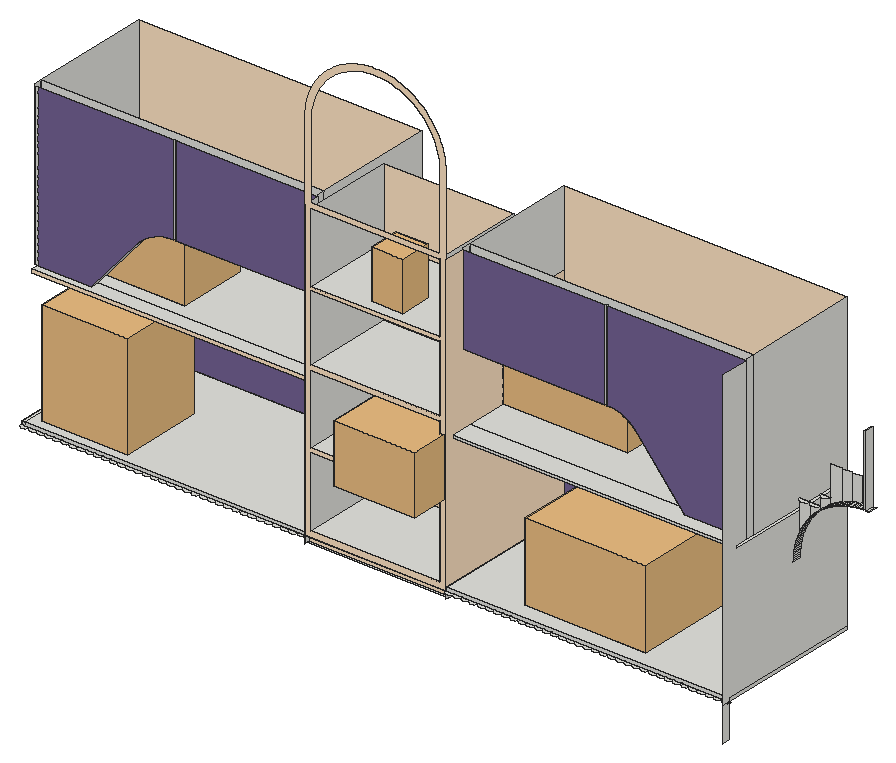
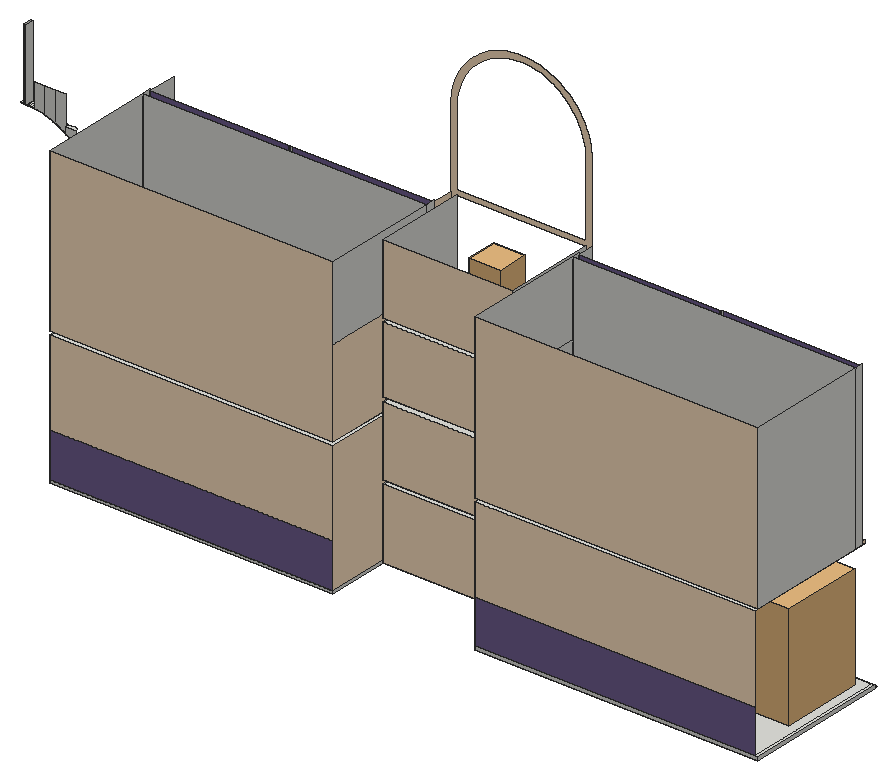
# SketchUp Ruby script. Lengths in inches.
U = 1.inch
M = Sketchup.active_model
def pt(a) = Geom::Point3d.new(a.map { |v| v * U })
def face(e, loops, mat)
  f = e.add_face(loops[0].map { |a| pt(a) })
  loops[1..].each { |l| e.add_face(l.map { |a| pt(a) }).erase! }
  f.material = f.back_material = mat if mat
  f
end
# faces: each face lists its corners as indices into pts; further lists are holes
def faces(e, pts, list, mat = nil) = list.each { |f| face(e, (f[0].is_a?(Array) ? f : [f]).map { |l| l.map { |i| pts[i] } }, mat) }
# xy, xz, yz: faces in a plane at the given z, y or x. An outline is a flat list of corners, or four numbers for a rectangle; further outlines are holes
def ring(l) = l.size == 4 ? [[l[0], l[1]], [l[2], l[1]], [l[2], l[3]], [l[0], l[3]]] : l.each_slice(2).to_a
def flat(e, list, mat, &to3) = list.each { |f| face(e, (f[0].is_a?(Array) ? f : [f]).map { |l| ring(l).map { |u, v| to3.(u, v) } }, mat) }
def xy(e, z, list, mat = nil) = flat(e, list, mat) { |x, y| [x, y, z] }
def xz(e, y, list, mat = nil) = flat(e, list, mat) { |x, z| [x, y, z] }
def yz(e, x, list, mat = nil) = flat(e, list, mat) { |y, z| [x, y, z] }
def lines(e, pts, list) = list.each { |a, b| e.add_line(pt(pts[a]), pt(pts[b])) }
# prism: a flat outline (further loops are holes) pulled along v
def prism(e, loops, v, mat = nil)
  f = face(e, loops, mat); d = Geom::Vector3d.new(v.map { |x| x * U })
  f.pushpull(f.normal.samedirection?(d) ? d.length : -d.length)
end
def box(e, o, s, mat = nil) = prism(e, [[o, [o[0] + s[0], o[1], o[2]], [o[0] + s[0], o[1] + s[1], o[2]], [o[0], o[1] + s[1], o[2]]]], [0, 0, s[2]], mat)
def at(x, y, z, deg = 0) = Geom::Transformation.translation(pt([x, y, z])) * Geom::Transformation.rotation(ORIGIN, Z_AXIS, deg.degrees)
def axes(o, x, y, z) = Geom::Transformation.new([*x, 0, *y, 0, *z, 0, *pt(o).to_a, 1])
def part(name) = M.definitions.add(name)
# library, detail: a bought-in or finely detailed component or shape, given as its bounding box
def library(name, o, s) = part(name).tap { |d| box(d.entities, o, s) }
def detail(e, o, s) = box(e.add_group.entities, o, s)
def put(e, d, t, mat = nil) = e.add_instance(d, t).tap { |i| i.material = mat if mat }
def group(e, t, mat = nil) = e.add_group.tap { |g| g.transformation = t; g.material = mat if mat }.entities
root = M.entities
M.materials.add("[0012_Bisque]").color = [255, 228, 196]
M.materials.add("[Color I01]").color = [116, 98, 147]
c1 = library("Flower+Vase+Glass",[1.07,1.25,0],[13.84,13.38,16.78])
c2 = library("Architecture and design books\#1",[9.67,-0.02,0],[20.02,11.1,12.25])
c3 = library("Group\#3",[0,0,0],[2.77,2.73,4.26])
c4 = library("pen_stand",[0,-5.91,0],[13.07,11.82,9.49])
c5 = library("LapTop",[-9.12,-3.35,-0.68],[14.19,15.07,9.17])
xy(root,39.45,[[50.74,141.7,73.56,142.13]])
xy(root,40.6875,[[5.77,140.54,5.94,140.5625,6.1,140.63,6.24,140.73,6.34,140.87,6.41,141.03,6.43,141.2,5.12,141.2,5.14,141.03,5.2,140.87,5.31,140.73,5.44,140.63,5.6,140.5625],[7.08,140.54,7.25,140.5625,7.41,140.63,7.55,140.73,7.65,140.87,7.72,141.03,7.74,141.2,6.43,141.2,6.45,141.03,6.52,140.87,6.62,140.73,6.76,140.63,6.91,140.5625],[8.4,140.54,8.57,140.5625,8.72,140.63,8.86,140.73,8.96,140.87,9.03,141.03,9.05,141.2,7.74,141.2,7.76,141.03,7.83,140.87,7.93,140.73,8.07,140.63,8.23,140.5625],[9.71,140.54,9.88,140.5625,10.04,140.63,10.17,140.73,10.28,140.87,10.34,141.03,10.37,141.2,9.05,141.2,9.08,141.03,9.14,140.87,9.24,140.73,9.38,140.63,9.54,140.5625],[11.02,140.54,11.19,140.5625,11.35,140.63,11.49,140.73,11.59,140.87,11.66,141.03,11.68,141.2,10.37,141.2,10.39,141.03,10.45,140.87,10.56,140.73,10.69,140.63,10.85,140.5625],
  [12.33,140.54,12.5,140.5625,12.66,140.63,12.8,140.73,12.9,140.87,12.97,141.03,12.99,141.2,11.68,141.2,11.7,141.03,11.77,140.87,11.87,140.73,12.01,140.63,12.16,140.5625],[13.65,140.54,13.82,140.5625,13.97,140.63,14.11,140.73,14.21,140.87,14.28,141.03,14.3,141.2,12.99,141.2,13.01,141.03,13.08,140.87,13.18,140.73,13.32,140.63,13.48,140.5625],[14.96,140.54,15.13,140.5625,15.29,140.63,15.42,140.73,15.53,140.87,15.59,141.03,15.62,141.2,14.3,141.2,14.33,141.03,14.39,140.87,14.49,140.73,14.63,140.63,14.79,140.5625],[16.27,140.54,16.44,140.5625,16.6,140.63,16.74,140.73,16.84,140.87,16.91,141.03,16.93,141.2,15.62,141.2,15.64,141.03,15.7,140.87,15.81,140.73,15.94,140.63,16.1,140.5625],[17.58,140.54,17.75,140.5625,17.91,140.63,18.05,140.73,18.15,140.87,18.22,141.03,18.24,141.2,16.93,141.2,16.95,141.03,17.02,140.87,17.12,140.73,17.26,140.63,17.41,140.5625],
  [18.9,140.54,19.07,140.5625,19.22,140.63,19.36,140.73,19.46,140.87,19.53,141.03,19.55,141.2,18.24,141.2,18.26,141.03,18.33,140.87,18.43,140.73,18.57,140.63,18.73,140.5625],[20.21,140.54,20.38,140.5625,20.54,140.63,20.67,140.73,20.78,140.87,20.84,141.03,20.87,141.2,19.55,141.2,19.58,141.03,19.64,140.87,19.74,140.73,19.88,140.63,20.04,140.5625],[21.52,140.54,21.69,140.5625,21.85,140.63,21.99,140.73,22.09,140.87,22.16,141.03,22.18,141.2,20.87,141.2,20.89,141.03,20.95,140.87,21.06,140.73,21.19,140.63,21.35,140.5625],[22.83,140.54,23,140.5625,23.16,140.63,23.3,140.73,23.4,140.87,23.47,141.03,23.49,141.2,22.18,141.2,22.2,141.03,22.27,140.87,22.37,140.73,22.51,140.63,22.66,140.5625],[24.15,140.54,24.32,140.5625,24.47,140.63,24.61,140.73,24.71,140.87,24.78,141.03,24.8,141.2,23.49,141.2,23.51,141.03,23.58,140.87,23.68,140.73,23.82,140.63,23.98,140.5625],
  [25.46,140.54,25.63,140.5625,25.79,140.63,25.92,140.73,26.03,140.87,26.09,141.03,26.12,141.2,24.8,141.2,24.83,141.03,24.89,140.87,24.99,140.73,25.13,140.63,25.29,140.5625],[26.77,140.54,26.94,140.5625,27.1,140.63,27.24,140.73,27.34,140.87,27.41,141.03,27.43,141.2,26.12,141.2,26.14,141.03,26.2,140.87,26.31,140.73,26.44,140.63,26.6,140.5625],[28.08,140.54,28.25,140.5625,28.41,140.63,28.55,140.73,28.65,140.87,28.72,141.03,28.74,141.2,27.43,141.2,27.45,141.03,27.52,140.87,27.62,140.73,27.76,140.63,27.91,140.5625],[29.4,140.54,29.57,140.5625,29.72,140.63,29.86,140.73,29.96,140.87,30.03,141.03,30.05,141.2,28.74,141.2,28.76,141.03,28.83,140.87,28.93,140.73,29.07,140.63,29.23,140.5625],[30.71,140.54,30.88,140.5625,31.04,140.63,31.17,140.73,31.28,140.87,31.34,141.03,31.37,141.2,30.05,141.2,30.08,141.03,30.14,140.87,30.24,140.73,30.38,140.63,30.54,140.5625],
  [32.02,140.54,32.19,140.5625,32.35,140.63,32.49,140.73,32.59,140.87,32.66,141.03,32.68,141.2,31.37,141.2,31.39,141.03,31.45,140.87,31.56,140.73,31.69,140.63,31.85,140.5625],[33.33,140.54,33.5,140.5625,33.66,140.63,33.8,140.73,33.9,140.87,33.97,141.03,33.99,141.2,32.68,141.2,32.7,141.03,32.77,140.87,32.87,140.73,33.01,140.63,33.16,140.5625],[34.65,140.54,34.82,140.5625,34.97,140.63,35.11,140.73,35.21,140.87,35.28,141.03,35.3,141.2,33.99,141.2,34.01,141.03,34.08,140.87,34.18,140.73,34.32,140.63,34.48,140.5625],[35.96,140.54,36.13,140.5625,36.29,140.63,36.42,140.73,36.53,140.87,36.59,141.03,36.62,141.2,35.3,141.2,35.33,141.03,35.39,140.87,35.49,140.73,35.63,140.63,35.79,140.5625],[37.27,140.54,37.44,140.5625,37.6,140.63,37.74,140.73,37.84,140.87,37.91,141.03,37.93,141.2,36.62,141.2,36.64,141.03,36.7,140.87,36.81,140.73,36.94,140.63,37.1,140.5625],
  [38.58,140.54,38.75,140.5625,38.91,140.63,39.05,140.73,39.15,140.87,39.22,141.03,39.24,141.2,37.93,141.2,37.95,141.03,38.02,140.87,38.12,140.73,38.26,140.63,38.41,140.5625],[39.9,140.54,40.07,140.5625,40.22,140.63,40.36,140.73,40.46,140.87,40.53,141.03,40.55,141.2,39.24,141.2,39.26,141.03,39.33,140.87,39.43,140.73,39.57,140.63,39.73,140.5625],[41.21,140.54,41.38,140.5625,41.54,140.63,41.67,140.73,41.78,140.87,41.84,141.03,41.87,141.2,40.55,141.2,40.58,141.03,40.64,140.87,40.74,140.73,40.88,140.63,41.04,140.5625],[42.52,140.54,42.69,140.5625,42.85,140.63,42.99,140.73,43.09,140.87,43.16,141.03,43.18,141.2,41.87,141.2,41.89,141.03,41.95,140.87,42.06,140.73,42.19,140.63,42.35,140.5625],[43.83,140.54,44,140.5625,44.16,140.63,44.3,140.73,44.4,140.87,44.47,141.03,44.49,141.2,43.18,141.2,43.2,141.03,43.27,140.87,43.37,140.73,43.51,140.63,43.66,140.5625],
  [45.15,140.54,45.32,140.5625,45.47,140.63,45.61,140.73,45.71,140.87,45.78,141.03,45.8,141.2,44.49,141.2,44.51,141.03,44.58,140.87,44.68,140.73,44.82,140.63,44.98,140.5625],[46.46,140.54,46.63,140.5625,46.79,140.63,46.92,140.73,47.03,140.87,47.09,141.03,47.12,141.2,45.8,141.2,45.83,141.03,45.89,140.87,45.99,140.73,46.13,140.63,46.29,140.5625],[47.77,140.54,47.94,140.5625,48.1,140.63,48.24,140.73,48.34,140.87,48.41,141.03,48.43,141.2,47.12,141.2,47.14,141.03,47.2,140.87,47.31,140.73,47.44,140.63,47.6,140.5625],[49.08,140.54,49.25,140.5625,49.41,140.63,49.55,140.73,49.65,140.87,49.72,141.03,49.74,141.2,48.43,141.2,48.45,141.03,48.52,140.87,48.62,140.73,48.76,140.63,48.91,140.5625],[74.21,140.54,74.38,140.5625,74.54,140.63,74.68,140.73,74.78,140.87,74.85,141.03,74.87,141.2,73.56,141.2,73.58,141.03,73.65,140.87,73.75,140.73,73.89,140.63,74.05,140.5625],
  [75.53,140.54,75.7,140.5625,75.86,140.63,75.99,140.73,76.1,140.87,76.16,141.03,76.18,141.2,74.87,141.2,74.89,141.03,74.96,140.87,75.0625,140.73,75.2,140.63,75.36,140.5625],[76.84,140.54,77.01,140.5625,77.17,140.63,77.3,140.73,77.41,140.87,77.47,141.03,77.5,141.2,76.18,141.2,76.21,141.03,76.27,140.87,76.375,140.73,76.51,140.63,76.67,140.5625],[78.15,140.54,78.32,140.5625,78.48,140.63,78.62,140.73,78.72,140.87,78.79,141.03,78.81,141.2,77.5,141.2,77.52,141.03,77.58,140.87,77.6875,140.73,77.82,140.63,77.98,140.5625],[79.46,140.54,79.63,140.5625,79.79,140.63,79.93,140.73,80.03,140.87,80.1,141.03,80.12,141.2,78.81,141.2,78.83,141.03,78.9,140.87,79,140.73,79.14,140.63,79.3,140.5625],[80.78,140.54,80.95,140.5625,81.11,140.63,81.24,140.73,81.35,140.87,81.41,141.03,81.43,141.2,80.12,141.2,80.14,141.03,80.21,140.87,80.3125,140.73,80.45,140.63,80.61,140.5625],
  [82.09,140.54,82.26,140.5625,82.42,140.63,82.55,140.73,82.66,140.87,82.72,141.03,82.75,141.2,81.43,141.2,81.46,141.03,81.52,140.87,81.625,140.73,81.76,140.63,81.92,140.5625],[83.4,140.54,83.57,140.5625,83.73,140.63,83.87,140.73,83.97,140.87,84.04,141.03,84.06,141.2,82.75,141.2,82.77,141.03,82.83,140.87,82.9375,140.73,83.07,140.63,83.23,140.5625],[84.71,140.54,84.88,140.5625,85.04,140.63,85.18,140.73,85.28,140.87,85.35,141.03,85.37,141.2,84.06,141.2,84.08,141.03,84.15,140.87,84.25,140.73,84.39,140.63,84.55,140.5625],[86.03,140.54,86.2,140.5625,86.36,140.63,86.49,140.73,86.6,140.87,86.66,141.03,86.68,141.2,85.37,141.2,85.39,141.03,85.46,140.87,85.5625,140.73,85.7,140.63,85.86,140.5625],[87.34,140.54,87.51,140.5625,87.67,140.63,87.8,140.73,87.91,140.87,87.97,141.03,88,141.2,86.68,141.2,86.71,141.03,86.77,140.87,86.875,140.73,87.01,140.63,87.17,140.5625],
  [88.65,140.54,88.82,140.5625,88.98,140.63,89.12,140.73,89.22,140.87,89.29,141.03,89.31,141.2,88,141.2,88.02,141.03,88.08,140.87,88.1875,140.73,88.32,140.63,88.48,140.5625],[89.96,140.54,90.13,140.5625,90.29,140.63,90.43,140.73,90.53,140.87,90.6,141.03,90.62,141.2,89.31,141.2,89.33,141.03,89.4,140.87,89.5,140.73,89.64,140.63,89.8,140.5625],[91.28,140.54,91.45,140.5625,91.61,140.63,91.74,140.73,91.85,140.87,91.91,141.03,91.93,141.2,90.62,141.2,90.64,141.03,90.71,140.87,90.8125,140.73,90.95,140.63,91.11,140.5625],[92.59,140.54,92.76,140.5625,92.92,140.63,93.05,140.73,93.16,140.87,93.22,141.03,93.25,141.2,91.93,141.2,91.96,141.03,92.02,140.87,92.125,140.73,92.26,140.63,92.42,140.5625],[93.9,140.54,94.07,140.5625,94.23,140.63,94.37,140.73,94.47,140.87,94.54,141.03,94.56,141.2,93.25,141.2,93.27,141.03,93.33,140.87,93.4375,140.73,93.57,140.63,93.73,140.5625],
  [95.21,140.54,95.38,140.5625,95.54,140.63,95.68,140.73,95.78,140.87,95.85,141.03,95.87,141.2,94.56,141.2,94.58,141.03,94.65,140.87,94.75,140.73,94.89,140.63,95.05,140.5625],[96.53,140.54,96.7,140.5625,96.86,140.63,96.99,140.73,97.1,140.87,97.16,141.03,97.18,141.2,95.87,141.2,95.89,141.03,95.96,140.87,96.0625,140.73,96.2,140.63,96.36,140.5625],[97.84,140.54,98.01,140.5625,98.17,140.63,98.3,140.73,98.41,140.87,98.47,141.03,98.5,141.2,97.18,141.2,97.21,141.03,97.27,140.87,97.375,140.73,97.51,140.63,97.67,140.5625],[99.15,140.54,99.32,140.5625,99.48,140.63,99.62,140.73,99.72,140.87,99.79,141.03,99.81,141.2,98.5,141.2,98.52,141.03,98.58,140.87,98.6875,140.73,98.82,140.63,98.98,140.5625],[100.46,140.54,100.63,140.5625,100.79,140.63,100.93,140.73,101.03,140.87,101.1,141.03,101.12,141.2,99.81,141.2,99.83,141.03,99.9,140.87,100,140.73,100.14,140.63,100.3,140.5625],
  [101.78,140.54,101.95,140.5625,102.11,140.63,102.24,140.73,102.35,140.87,102.41,141.03,102.43,141.2,101.12,141.2,101.14,141.03,101.21,140.87,101.3125,140.73,101.45,140.63,101.61,140.5625],[103.09,140.54,103.26,140.5625,103.42,140.63,103.55,140.73,103.66,140.87,103.72,141.03,103.75,141.2,102.43,141.2,102.46,141.03,102.52,140.87,102.625,140.73,102.76,140.63,102.92,140.5625],[104.4,140.54,104.57,140.5625,104.73,140.63,104.87,140.73,104.97,140.87,105.04,141.03,105.06,141.2,103.75,141.2,103.77,141.03,103.83,140.87,103.9375,140.73,104.07,140.63,104.23,140.5625],[105.71,140.54,105.88,140.5625,106.04,140.63,106.18,140.73,106.28,140.87,106.35,141.03,106.37,141.2,105.06,141.2,105.08,141.03,105.15,140.87,105.25,140.73,105.39,140.63,105.55,140.5625],[107.03,140.54,107.2,140.5625,107.36,140.63,107.49,140.73,107.6,140.87,107.66,141.03,107.68,141.2,106.37,141.2,106.39,141.03,106.46,140.87,106.5625,140.73,106.7,140.63,106.86,140.5625],
  [108.34,140.54,108.51,140.5625,108.67,140.63,108.8,140.73,108.91,140.87,108.97,141.03,109,141.2,107.68,141.2,107.71,141.03,107.77,140.87,107.875,140.73,108.01,140.63,108.17,140.5625],[109.65,140.54,109.82,140.5625,109.98,140.63,110.12,140.73,110.22,140.87,110.29,141.03,110.31,141.2,109,141.2,109.02,141.03,109.08,140.87,109.1875,140.73,109.32,140.63,109.48,140.5625],[110.96,140.54,111.13,140.5625,111.29,140.63,111.43,140.73,111.53,140.87,111.6,141.03,111.62,141.2,110.31,141.2,110.33,141.03,110.4,140.87,110.5,140.73,110.64,140.63,110.8,140.5625],[112.28,140.54,112.45,140.5625,112.61,140.63,112.74,140.73,112.85,140.87,112.91,141.03,112.93,141.2,111.62,141.2,111.64,141.03,111.71,140.87,111.8125,140.73,111.95,140.63,112.11,140.5625],[113.59,140.54,113.76,140.5625,113.92,140.63,114.05,140.73,114.16,140.87,114.22,141.03,114.25,141.2,112.93,141.2,112.96,141.03,113.02,140.87,113.125,140.73,113.26,140.63,113.42,140.5625],
  [114.9,140.54,115.07,140.5625,115.23,140.63,115.37,140.73,115.47,140.87,115.54,141.03,115.56,141.2,114.25,141.2,114.27,141.03,114.33,140.87,114.4375,140.73,114.57,140.63,114.73,140.5625],[116.21,140.54,116.38,140.5625,116.54,140.63,116.68,140.73,116.78,140.87,116.85,141.03,116.87,141.2,115.56,141.2,115.58,141.03,115.65,140.87,115.75,140.73,115.89,140.63,116.05,140.5625],[117.53,140.54,117.7,140.5625,117.86,140.63,117.99,140.73,118.1,140.87,118.16,141.03,118.18,141.2,116.87,141.2,116.89,141.03,116.96,140.87,117.0625,140.73,117.2,140.63,117.36,140.5625],[118.84,140.54,119.01,140.5625,119.17,140.63,119.1875,140.64,119.1875,141.2,118.18,141.2,118.21,141.03,118.27,140.87,118.375,140.73,118.51,140.63,118.67,140.5625],[119.1875,140.64,119.3,140.73,119.41,140.87,119.47,141.03,119.5,141.2,119.1875,141.2],
  [50.375,140.71,50.54,140.73,50.7,140.8,50.84,140.9,50.94,141.04,51.01,141.2,49.74,141.2,49.81,141.04,49.91,140.9,50.05,140.8,50.2,140.73],[5.12,141.2,50.74,164.88],[50.74,141.2,51.01,141.2,51.03,141.37,50.74,141.37],[51.01,141.2,51.03,141.37,50.74,141.37,50.74,142.13,73.56,142.13,73.56,141.2],[73.56,141.2,119.1875,164.88]])
xy(root,41.1875,[[5.12,141.2,5.62,164.88],[5.62,141.2,50.74,164.88],[73.56,141.2,119.1875,164.88]])
xy(root,41.64,[[51.69,141.2,72.61,155.95]])
xy(root,52.99,[[51.69,141.2,72.61,155.95]])
xy(root,53.64,[[51.69,141.2,72.61,155.95]])
xy(root,62.0625,[[5.62,142.63,50.74,164.88],[73.56,142.63,119.1875,164.88]])
xy(root,62.625,[[5.62,142.63,50.74,142.63,50.74,145.09,14.3,145.09,14.3,143.84,5.62,143.84],[73.56,142.63,119.1875,142.63,119.1875,144.68,109.19,144.68,109.19,146.09,73.56,146.09],[5.12,143.84,14.3,145.09],[109.19,144.68,119.1875,146.09],[5.12,145.09,50.74,164.88],
  [73.56,146.09,119.1875,164.88]])
xy(root,64.86,[[51.69,141.2,72.61,155.95]])
xy(root,65.64,[[51.69,141.2,72.61,155.95]])
xy(root,74.0625,[[27.93,143.84,27.93,144.02,27.56,144.02,27.56,145.09,50.74,145.09,50.74,143.84],[73.56,144.68,73.56,146.09,96.75,146.09,96.75,144.86,96.375,144.86,96.375,144.68]])
xy(root,74.15,[[131.36,140.54,131.52,140.54,131.59,140.55,131.67,140.57,131.74,140.59,131.88,140.66,131.94,140.7,132.06,140.8,132.16,140.92,132.2,140.98,132.23,141.05,132.26,141.125,132.28,141.2,130.59,141.2,130.65,141.05,130.68,140.98,130.72,140.92,130.82,140.8,130.93,140.7,131,140.66,131.14,140.59,131.21,140.57,131.29,140.55],[133.05,140.54,133.2,140.54,133.28,140.55,133.35,140.57,133.43,140.59,133.57,140.66,133.63,140.7,133.75,140.8,133.8,140.86,133.88,140.98,133.92,141.05,133.95,141.125,133.97,141.2,132.28,141.2,132.3,141.125,132.33,141.05,132.37,140.98,132.45,140.86,132.51,140.8,132.5625,140.75,132.62,140.7,132.6875,140.66,132.75,140.625,132.83,140.59,132.97,140.55]])
xy(root,75.9375,[[134.74,140.54,134.89,140.54,134.97,140.55,135.11,140.59,135.25,140.66,135.32,140.7,135.38,140.75,135.49,140.86,135.57,140.98,135.61,141.05,135.64,141.125,135.66,141.2,133.97,141.2,133.99,141.125,134.02,141.05,134.06,140.98,134.14,140.86,134.19,140.8,134.31,140.7,134.375,140.66,134.44,140.625,134.51,140.59,134.59,140.57,134.66,140.55]])
xy(root,76.42,[[51.69,141.2,72.61,155.95]])
xy(root,76.87,[[141.32,140.59,141.48,140.62,141.63,140.68,141.77,140.78,141.875,140.9,141.96,141.04,142,141.2,140.59,141.2,140.57,141.125,140.5625,141.1,140.63,140.95,140.73,140.82,140.85,140.71,141,140.64,141.16,140.6]])
xy(root,76.95,[[51.69,141.2,72.61,155.95]])
xy(root,76.97,[[142.3,139.88,142.31,141.2]])
xz(root,141.2,[[5.12,40.6875,5.62,41.1875],[5.62,40.6875,50.74,41.1875],[73.56,40.6875,119.1875,41.1875],[130.59,65.41,130.59,74.15,132.28,74.15,132.28,71.42,132.27,71.4,132.12,71.15,131.97,70.88,131.83,70.62,131.7,70.35,131.58,70.07,131.46,69.8,131.35,69.52,131.25,69.24,131.15,68.95,131.0625,68.67,130.98,68.38,130.91,68.09,130.84,67.79,130.79,67.5,130.73,67.2,130.69,66.91,130.63,66.31,130.61,66.01],[132.28,71.42,132.28,74.15,133.97,74.15,133.97,73.57,133.93,73.53,133.72,73.3125,133.52,73.09,133.32,72.87,133.13,72.63,132.94,72.4,132.77,72.16,132.59,71.91,132.43,71.66],
  [133.97,73.57,133.97,75.9375,135.66,75.9375,135.66,74.97,135.53,74.88,135.29,74.71,135.05,74.53,134.8125,74.34,134.58,74.15,134.36,73.95,134.14,73.74],[135.66,74.97,135.66,80.75,137.28,80.75,137.28,75.89,137.08,75.8,136.8125,75.66,136.55,75.52,136.03,75.22,135.78,75.05],[137.34,75.92,137.34,80.75,138.91,80.75,138.91,76.5,138.75,76.46,138.47,76.37,138.18,76.27,137.9,76.16,137.625,76.05,137.35,75.93],[138.97,76.52,138.97,80.75,140.53,80.75,140.53,76.86,140.51,76.85,140.21,76.81,139.92,76.75,139.62,76.69,139.33,76.62,139.04,76.54],[142,76.95,142.3,76.97,142.3,88.4375,142,88.4375]])
xz(root,141.2,[[[50.74,40.6875,73.56,40.6875,73.56,100.6875,73.54,101.28,73.5,101.88,73.42,102.47,73.31,103.06,73.17,103.64,73,104.21,72.8,104.78,72.57,105.33,72.32,105.87,72.03,106.39,71.72,106.9,71.38,107.39,71.02,107.87,70.63,108.32,70.22,108.75,69.78,109.16,69.33,109.55,68.86,109.92,68.36,110.25,67.85,110.57,67.33,110.85,66.79,111.11,66.24,111.34,65.68,111.54,65.1,111.71,64.52,111.85,63.9375,111.95,63.34,112.03,62.75,112.08,62.15,112.09,61.55,112.08,60.96,112.03,60.37,111.95,59.78,111.85,59.2,111.71,58.625,111.54,58.0625,111.34,57.51,111.11,56.97,110.85,56.45,110.57,55.9375,110.25,55.45,109.92,54.97,109.55,54.52,109.16,54.09,108.75,53.67,108.32,53.29,107.87,52.92,107.39,52.58,106.9,52.27,106.39,51.99,105.87,51.73,105.33,51.5,104.78,51.3,104.21,51.13,103.64,50.99,103.06,50.88,102.47,50.81,101.88,50.76,101.28,50.74,100.6875],[51.69,88.95,51.69,100.6875,51.71,101.23,51.75,101.78,51.82,102.32,51.92,102.86,52.05,103.39,52.21,103.92,52.39,104.43,52.6,104.94,52.83,105.43,53.1,105.92,53.38,106.38,53.69,106.83,54.02,107.27,54.38,107.68,54.76,108.08,55.15,108.46,55.57,108.8125,56,109.15,56.46,109.46,56.92,109.74,57.4,110,57.9,110.24,58.4,110.45,58.92,110.63,59.44,110.79,59.98,110.92,60.52,111.02,61.06,111.09,61.6,111.13,62.15,111.14,62.7,111.13,63.24,111.09,63.79,111.02,64.33,110.92,64.86,110.79,65.38,110.63,65.9,110.45,66.4,110.24,66.9,110,67.38,109.74,67.85,109.46,68.3,109.15,68.73,108.8125,69.15,108.46,69.55,108.08,69.92,107.68,70.28,107.27,70.61,106.83,70.92,106.38,71.21,105.92,71.47,105.43,71.7,104.94,71.91,104.43,72.1,103.92,72.25,103.39,72.38,102.86,72.48,102.32,72.55,101.78,72.59,101.23,72.61,100.6875,72.61,88.95],[51.69,41.64,72.61,52.99],[51.69,76.95,72.61,88.24],[51.69,53.64,72.61,64.86],[51.69,65.64,72.61,76.42]]],"[0012_Bisque]")
xz(root,142.13,[[50.74,39.45,73.56,40.6875]],"[0012_Bisque]")
xz(root,142.63,[[73.56,62.0625,119.1875,62.625]])
xz(root,142.63,[[5.62,62.0625,50.74,62.625]],"[0012_Bisque]")
xz(root,143.84,[[5.12,62.625,5.62,88.4375]])
xz(root,143.84,[[5.62,62.625,14.3,62.625,21.76,71.45,22.13,71.86,22.53,72.23,22.95,72.58,23.4,72.89,23.875,73.17,24.36,73.42,24.87,73.62,25.39,73.79,25.92,73.92,26.46,74.01,27.01,74.05,27.56,74.0625,27.56,88.4375,5.62,88.4375],[27.93,74.0625,50.74,88.4375]],"[Color I01]")
xz(root,144.02,[[27.56,74.0625,27.93,88.4375]])
xz(root,144.68,[[109.19,62.625,119.1875,62.625,119.1875,88.4375,96.75,88.4375,96.75,74.0625,97.22,74.04,97.6875,73.99,98.15,73.9,98.6,73.77,99.05,73.61,99.47,73.41,99.89,73.1875,100.28,72.93,100.65,72.64,101,72.32,101.32,71.98,101.62,71.61],[73.56,74.0625,96.375,88.4375]],"[Color I01]")
xz(root,144.86,[[96.375,74.0625,96.75,88.4375]])
xz(root,145.09,[[5.12,62.625,5.12,88.6875,50.74,88.6875,50.74,74.0625,27.56,74.0625,27.01,74.05,26.46,74.01,25.92,73.92,25.39,73.79,24.87,73.62,24.36,73.42,23.875,73.17,23.4,72.89,22.95,72.58,22.53,72.23,22.13,71.86,21.76,71.45,14.3,62.625]])
xz(root,146.09,[[109.19,62.625,101.62,71.61,101.32,71.98,101,72.32,100.65,72.64,100.28,72.93,99.89,73.1875,99.47,73.41,99.05,73.61,98.6,73.77,98.15,73.9,97.6875,73.99,97.22,74.04,96.75,74.0625,73.56,74.0625,73.56,88.6875,119.1875,88.6875,119.1875,62.625]])
xz(root,155.95,[[51.69,41.64,72.61,52.99],[51.69,53.64,72.61,64.86],[51.69,65.64,72.61,76.42],[51.69,76.95,72.61,88.24]],"[0012_Bisque]")
xz(root,164.88,[[5.12,40.6875,50.74,41.1875],[73.56,40.6875,119.1875,41.1875]])
xz(root,164.88,[[5.62,48.3125,50.74,62.0625],[73.56,48.3125,119.1875,62.0625],[5.12,62.625,50.74,88.6875],[73.56,62.625,119.1875,88.6875]],"[0012_Bisque]")
xz(root,164.88,[[5.62,41.1875,50.74,48.3125],[73.56,41.1875,119.1875,48.3125]],"[Color I01]")
yz(root,5.12,[[141.2,40.6875,164.88,41.1875],[143.84,62.625,145.09,88.6875],[145.09,62.625,164.88,88.6875]])
yz(root,27.56,[[143.84,74.0625,144.02,88.4375]])
yz(root,27.93,[[143.84,74.0625,144.02,88.4375]])
yz(root,50.74,[[141.2,39.45,141.37,40.6875],[141.37,39.45,142.13,40.6875],[141.2,40.6875,142.13,41.1875],[142.13,40.6875,164.88,41.1875],[141.2,41.1875,141.2,88.4375,143.84,88.4375,143.84,74.0625,145.09,74.0625,145.09,76.6875,164.88,76.6875,164.88,62.625,142.63,62.625,142.63,62.0625,164.88,62.0625,164.88,41.1875],
  [143.84,74.0625,145.09,76.6875],[143.84,76.6875,145.09,88.6875],[145.09,76.6875,164.88,88.6875]])
yz(root,51.69,[[141.2,41.64,155.95,52.99],[141.2,53.64,155.95,64.86],[141.2,65.64,155.95,76.42],[141.2,76.95,155.95,88.24]])
yz(root,72.61,[[141.2,41.64,155.95,52.99],[141.2,53.64,155.95,64.86],[141.2,65.64,155.95,76.42],[141.2,76.95,155.95,88.24]])
yz(root,73.56,[[141.2,39.45,142.13,40.6875],[141.2,40.6875,142.13,41.1875],[142.13,40.6875,164.88,41.1875],[144.68,74.0625,146.09,76.6875],[144.68,76.6875,146.09,88.6875],
  [146.09,76.6875,164.88,88.6875]])
yz(root,73.56,[[141.2,41.1875,164.88,41.1875,164.88,62.0625,142.63,62.0625,142.63,62.625,164.88,62.625,164.88,76.6875,146.09,76.6875,146.09,74.0625,144.68,74.0625,144.68,88.4375,141.2,88.4375]],"[0012_Bisque]")
yz(root,96.375,[[144.68,74.0625,144.86,88.4375]])
yz(root,96.75,[[144.68,74.0625,144.86,88.4375]])
yz(root,119.1875,[[139.88,35.18,141.2,40.6875],[139.88,40.6875,139.88,88.4375,144.68,88.4375,144.68,62.625,142.63,62.625,142.63,62.0625,164.88,62.0625,164.88,41.1875,141.2,41.1875,141.2,40.6875],[141.2,40.6875,164.88,41.1875],[144.68,62.625,146.09,88.6875],[146.09,62.625,164.88,88.6875]])
yz(root,142,[[139.88,76.95,141.2,88.4375]])
yz(root,142.3,[[139.88,76.97,141.2,88.4375]])
p = [[21.76,143.84,71.45],[14.3,143.84,62.625],[14.3,145.09,62.625],[21.76,145.09,71.45],[109.19,144.68,62.625],[101.62,144.68,71.61],
  [101.62,146.09,71.61],[109.19,146.09,62.625],[130.59,141.2,65.41],[130.6,141.2,65.71],[130.6,139.88,65.71],[130.59,139.88,65.41],
  [130.61,141.2,66.01],[130.61,139.88,66.01],[130.63,141.2,66.31],[130.63,139.88,66.31],[130.66,141.2,66.61],[130.66,139.88,66.61],
  [130.69,141.2,66.91],[130.69,139.88,66.91],[130.73,141.2,67.2],[130.73,139.88,67.2],[130.79,141.2,67.5],[130.79,139.88,67.5],
  [130.84,141.2,67.79],[130.84,139.88,67.79],[130.91,141.2,68.09],[130.91,139.88,68.09],[130.98,141.2,68.38],[130.98,139.88,68.38],
  [131.0625,141.2,68.67],[131.0625,139.88,68.67],[131.15,141.2,68.95],[131.15,139.88,68.95],[131.25,141.2,69.24],[131.25,139.88,69.24],
  [131.35,141.2,69.52],[131.35,139.88,69.52],[131.46,141.2,69.8],[131.46,139.88,69.8],[131.58,141.2,70.07],[131.58,139.88,70.07],
  [131.7,141.2,70.35],[131.7,139.88,70.35],[131.83,141.2,70.62],[131.83,139.88,70.62],[131.97,141.2,70.88],[131.97,139.88,70.88],
  [132.12,141.2,71.15],[132.12,139.88,71.15],[132.27,141.2,71.4],[132.27,139.88,71.4],[132.28,141.2,71.42],[132.43,141.2,71.66],
  [132.43,139.88,71.66],[22.13,143.84,71.86],[22.13,145.09,71.86],[101.32,144.68,71.98],[101.32,146.09,71.98],[132.59,141.2,71.91],
  [132.59,139.88,71.91],[132.77,141.2,72.16],[132.77,139.88,72.16],[22.53,143.84,72.23],[22.53,145.09,72.23],[101,144.68,72.32],
  [101,146.09,72.32],[132.94,141.2,72.4],[132.94,139.88,72.4],[22.95,143.84,72.58],[22.95,145.09,72.58],[100.65,144.68,72.64],
  [100.65,146.09,72.64],[133.13,141.2,72.63],[133.13,139.88,72.63],[133.32,141.2,72.87],[133.32,139.88,72.87],[23.4,143.84,72.89],
  [23.4,145.09,72.89],[100.28,144.68,72.93],[100.28,146.09,72.93],[133.52,141.2,73.09],[133.52,139.88,73.09],[23.875,143.84,73.17],
  [23.875,145.09,73.17],[99.89,144.68,73.1875],[99.89,146.09,73.1875],[133.72,141.2,73.3125],[133.72,139.88,73.3125],[24.36,143.84,73.42],
  [24.36,145.09,73.42],[99.47,144.68,73.41],[99.47,146.09,73.41],[133.93,141.2,73.53],[133.93,139.88,73.53],[24.87,143.84,73.62],
  [24.87,145.09,73.62],[99.05,144.68,73.61],[99.05,146.09,73.61],[133.97,141.2,73.57],[134.14,141.2,73.74],[134.14,139.88,73.74],
  [25.39,143.84,73.79],[25.39,145.09,73.79],[98.6,144.68,73.77],[98.6,146.09,73.77],[134.36,141.2,73.95],[134.36,139.88,73.95],
  [25.92,143.84,73.92],[25.92,145.09,73.92],[98.15,144.68,73.9],[98.15,146.09,73.9],[134.58,141.2,74.15],[134.58,139.88,74.15],
  [26.46,143.84,74.01],[26.46,145.09,74.01],[97.6875,144.68,73.99],[97.6875,146.09,73.99],[27.01,143.84,74.05],[27.01,145.09,74.05],
  [97.22,144.68,74.04],[96.75,144.68,74.0625],[96.75,144.86,74.0625],[96.75,146.09,74.0625],[97.22,146.09,74.04],[134.8125,141.2,74.34],
  [134.8125,139.88,74.34],[27.56,143.84,74.0625],[27.56,145.09,74.0625],[27.56,144.02,74.0625],[135.05,141.2,74.53],[135.05,139.88,74.53],
  [135.29,141.2,74.71],[135.29,139.88,74.71],[135.53,141.2,74.88],[135.53,139.88,74.88],[135.66,141.2,74.97],[135.78,141.2,75.05],
  [135.78,139.88,75.05],[136.03,141.2,75.22],[136.03,139.88,75.22],[136.29,141.2,75.37],[136.29,139.88,75.37],[136.55,141.2,75.52],
  [136.55,139.88,75.52],[136.8125,141.2,75.66],[136.8125,139.88,75.66],[137.08,141.2,75.8],[137.08,139.88,75.8],[137.28,141.2,75.89],
  [137.34,141.2,75.92],[137.35,141.2,75.93],[137.35,139.88,75.93],[137.625,141.2,76.05],[137.625,139.88,76.05],[137.9,141.2,76.16],
  [137.9,139.88,76.16],[138.18,141.2,76.27],[138.18,139.88,76.27],[138.47,141.2,76.37],[138.47,139.88,76.37],[138.75,141.2,76.46],
  [138.75,139.88,76.46],[138.91,141.2,76.5],[138.97,141.2,76.52],[139.04,141.2,76.54],[139.04,139.88,76.54],[139.33,141.2,76.62],
  [139.33,139.88,76.62],[139.62,141.2,76.69],[139.62,139.88,76.69],[139.92,141.2,76.75],[139.92,139.88,76.75],[140.21,141.2,76.81],
  [140.21,139.88,76.81],[140.51,141.2,76.85],[140.51,139.88,76.85],[140.53,141.2,76.86],[140.59,141.2,76.87],[140.8,141.2,76.89],
  [140.8,139.88,76.89],[141.1,141.2,76.92],[141.1,139.88,76.92],[141.4,141.2,76.95],[141.4,139.88,76.95],[141.7,141.2,76.96],
  [141.7,139.88,76.96],[142.61,141.2,76.96],[142.92,141.2,76.95],[142.92,139.88,76.95],[142.61,139.88,76.96],[142,141.2,76.95],
  [142,139.88,76.95],[142.31,141.2,76.97],[142.31,139.88,76.97],[51.01,141.2,39.45],[51.01,141.7,39.45]]
faces(root,p,[[0,1,2,3],[4,5,6,7],[8,9,10,11],[9,12,13,10],[12,14,15,13],[14,16,17,15],[16,18,19,17],[18,20,21,19],
  [20,22,23,21],[22,24,25,23],[24,26,27,25],[26,28,29,27],[28,30,31,29],[30,32,33,31],[32,34,35,33],[34,36,37,35],
  [36,38,39,37],[38,40,41,39],[40,42,43,41],[42,44,45,43],[44,46,47,45],[46,48,49,47],[48,50,51,49],[50,52,53,54,51],
  [55,0,3,56],[5,57,58,6],[53,59,60,54],[59,61,62,60],[63,55,56,64],[57,65,66,58],[61,67,68,62],[69,63,64,70],
  [65,71,72,66],[67,73,74,68],[73,75,76,74],[77,69,70,78],[71,79,80,72],[75,81,82,76],[83,77,78,84],[79,85,86,80],
  [81,87,88,82],[89,83,84,90],[85,91,92,86],[87,93,94,88],[95,89,90,96],[91,97,98,92],[93,99,100,101,94],[102,95,96,103],
  [97,104,105,98],[100,106,107,101],[108,102,103,109],[104,110,111,105],[106,112,113,107],[114,108,109,115],[110,116,117,111],[118,114,115,119],
  [120,121,122,123,124],[116,120,124,117],[112,125,126,113],[127,118,119,128,129],[125,130,131,126],[130,132,133,131],[132,134,135,133],[134,136,137,138,135],
  [137,139,140,138],[139,141,142,140],[141,143,144,142],[143,145,146,144],[145,147,148,146],[147,149,150,151,152,148],[151,153,154,152],[153,155,156,154],
  [155,157,158,156],[157,159,160,158],[159,161,162,160],[161,163,164,165,166,162],[165,167,168,166],[167,169,170,168],[169,171,172,170],[171,173,174,172],
  [173,175,176,174],[175,177,178,179,180,176],[179,181,182,180],[181,183,184,182],[183,185,186,184],[187,188,189,190],[185,191,192,186],[193,187,190,194]])
lines(root,p,[[195,196]])
put(root,c1,at(6.08,141.49,41.1875))
put(root,c2,at(-3.13,147.41,62.625))
put(root,c3,axes([60.05,143.04,76.95],[1.8328,0,0],[0,1.8328,0],[0,0,1.8328]))
put(root,c4,at(60.14,141.2,53.64))
put(root,c2,at(63.89,152.75,62.6))
put(root,c5,axes([96.73,148.4,42.125],[1.37,0,0],[0,1.37,0],[0,0,1.37]))
